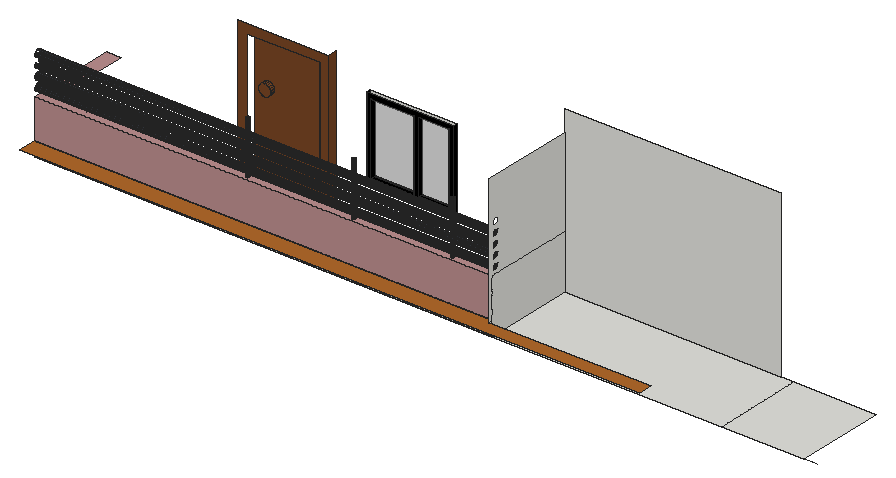
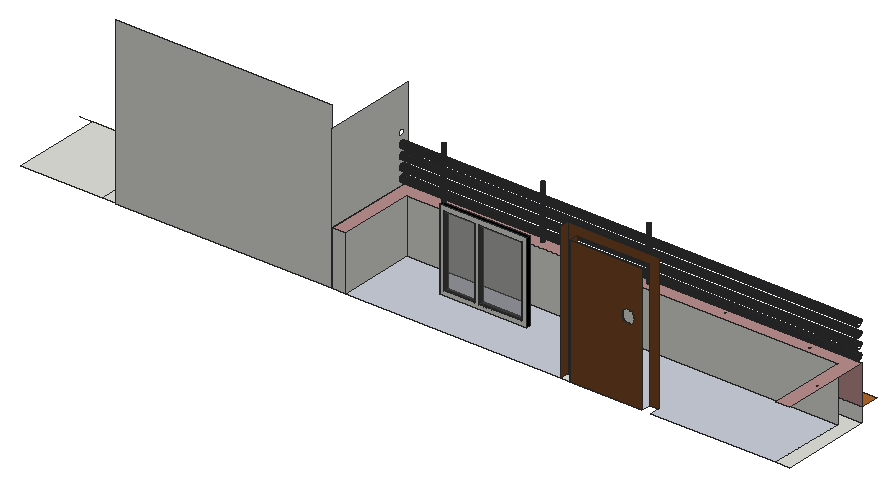
# SketchUp Ruby script. Lengths in inches.
U = 1.inch
M = Sketchup.active_model
def pt(a) = Geom::Point3d.new(a.map { |v| v * U })
def face(e, loops, mat)
  f = e.add_face(loops[0].map { |a| pt(a) })
  loops[1..].each { |l| e.add_face(l.map { |a| pt(a) }).erase! }
  f.material = f.back_material = mat if mat
  f
end
# faces: each face lists its corners as indices into pts; further lists are holes
def faces(e, pts, list, mat = nil) = list.each { |f| face(e, (f[0].is_a?(Array) ? f : [f]).map { |l| l.map { |i| pts[i] } }, mat) }
# xy, xz, yz: faces in a plane at the given z, y or x. An outline is a flat list of corners, or four numbers for a rectangle; further outlines are holes
def ring(l) = l.size == 4 ? [[l[0], l[1]], [l[2], l[1]], [l[2], l[3]], [l[0], l[3]]] : l.each_slice(2).to_a
def flat(e, list, mat, &to3) = list.each { |f| face(e, (f[0].is_a?(Array) ? f : [f]).map { |l| ring(l).map { |u, v| to3.(u, v) } }, mat) }
def xy(e, z, list, mat = nil) = flat(e, list, mat) { |x, y| [x, y, z] }
def xz(e, y, list, mat = nil) = flat(e, list, mat) { |x, z| [x, y, z] }
def yz(e, x, list, mat = nil) = flat(e, list, mat) { |y, z| [x, y, z] }
def lines(e, pts, list) = list.each { |a, b| e.add_line(pt(pts[a]), pt(pts[b])) }
# prism: a flat outline (further loops are holes) pulled along v
def prism(e, loops, v, mat = nil)
  f = face(e, loops, mat); d = Geom::Vector3d.new(v.map { |x| x * U })
  f.pushpull(f.normal.samedirection?(d) ? d.length : -d.length)
end
def box(e, o, s, mat = nil) = prism(e, [[o, [o[0] + s[0], o[1], o[2]], [o[0] + s[0], o[1] + s[1], o[2]], [o[0], o[1] + s[1], o[2]]]], [0, 0, s[2]], mat)
def at(x, y, z, deg = 0) = Geom::Transformation.translation(pt([x, y, z])) * Geom::Transformation.rotation(ORIGIN, Z_AXIS, deg.degrees)
def axes(o, x, y, z) = Geom::Transformation.new([*x, 0, *y, 0, *z, 0, *pt(o).to_a, 1])
def part(name) = M.definitions.add(name)
# library, detail: a bought-in or finely detailed component or shape, given as its bounding box
def library(name, o, s) = part(name).tap { |d| box(d.entities, o, s) }
def detail(e, o, s) = box(e.add_group.entities, o, s)
def put(e, d, t, mat = nil) = e.add_instance(d, t).tap { |i| i.material = mat if mat }
def group(e, t, mat = nil) = e.add_group.tap { |g| g.transformation = t; g.material = mat if mat }.entities
root = M.entities
M.materials.add("[0119_RosyBrown]").color = [188, 143, 143]
M.materials.add("[0137_Black]").color = [0, 0, 0]
M.materials.add("[Formica Laminate Dark]").color = [50, 53, 60]
M.materials.add("[Marble Carrara Floor Tile]").color = [204, 208, 219]
M.materials.add("[Translucent Glass Gray]").color = [128, 128, 128]
M.materials["[Translucent Glass Gray]"].alpha = 0.5
M.materials.add("[Wood Bamboo]").color = [177, 105, 43]
M.materials.add("[Wood Veneer 01]").color = [120, 70, 37]
xy(root,370.9,[[3.53,201.0625,3.53,261.0625,12.53,261.0625,12.53,210.0625,298.22,210.0625,298.22,261.0625,307.22,261.0625,307.22,201.0625],[307.22,201.0625,459.59,261.0625],[459.59,201.0625,514.15,261.0625],[149.3,255.0625,155.3,261.0625]])
xy(root,370.9,[[12.53,210.0625,298.22,210.0625,298.22,261.0625,155.3,261.0625,155.3,255.0625,149.3,255.0625,149.3,261.0625,101.3,261.0625,101.3,255.0625,95.3,255.0625,95.3,261.0625,12.53,261.0625]],"[Marble Carrara Floor Tile]")
xy(root,380.59,[[3.53,189.0625,414.72,189.0625,414.72,198.0625,307.22,198.0625,307.22,201.0625,3.53,201.0625]],"[Wood Bamboo]")
xy(root,392.51,[[178.09,258.0625,235.97,261.0625]])
xy(root,395.51,[[181.09,258.0625,209.84,261.0625],[212.72,258.0625,232.97,261.0625]],"[0137_Black]")
xy(root,406.9,[[142.52,203.04,142.26,203.07,142.02,203.17,141.81,203.33,141.65,203.54,141.55,203.78,141.52,204.04,141.55,204.3,141.65,204.54,141.81,204.75,142.02,204.91,142.26,205.01,142.52,205.04,142.78,205.01,143.02,204.91,143.22,204.75,143.38,204.54,143.48,204.3,143.52,204.04,143.48,203.78,143.38,203.54,143.22,203.33,143.02,203.17,142.78,203.07],[212.89,203.04,212.63,203.07,212.39,203.17,212.18,203.33,212.03,203.54,211.93,203.78,211.89,204.04,211.93,204.3,212.03,204.54,212.18,204.75,212.39,204.91,212.63,205.01,212.89,205.04,213.15,205.01,213.39,204.91,213.6,204.75,213.76,204.54,213.86,204.3,213.89,204.04,213.86,203.78,213.76,203.54,213.6,203.33,213.39,203.17,213.15,203.07]])
xy(root,406.9,[[[3.53,201.0625,307.22,201.0625,307.22,261.0625,298.22,261.0625,298.22,210.0625,12.53,210.0625,12.53,261.0625,3.53,261.0625],[34.52,204.5,34.26,204.53,34.02,204.63,33.82,204.79,33.66,205,33.56,205.24,33.52,205.5,33.56,205.76,33.66,206,33.82,206.21,34.02,206.37,34.26,206.47,34.52,206.5,34.78,206.47,35.02,206.37,35.23,206.21,35.39,206,35.49,205.76,35.52,205.5,35.49,205.24,35.39,205,35.23,204.79,35.02,204.63,34.78,204.53],[91.52,203.04,91.26,203.07,91.02,203.17,90.81,203.33,90.65,203.54,90.55,203.78,90.52,204.04,90.55,204.3,90.65,204.54,90.81,204.75,91.02,204.91,91.26,205.01,91.52,205.04,91.78,205.01,92.02,204.91,92.22,204.75,92.38,204.54,92.48,204.3,92.52,204.04,92.48,203.78,92.38,203.54,92.22,203.33,92.02,203.17,91.78,203.07],[142.52,203.04,142.26,203.07,142.02,203.17,141.81,203.33,141.65,203.54,141.55,203.78,141.52,204.04,141.55,204.3,141.65,204.54,141.81,204.75,142.02,204.91,142.26,205.01,142.52,205.04,142.78,205.01,143.02,204.91,143.22,204.75,143.38,204.54,143.48,204.3,143.52,204.04,143.48,203.78,143.38,203.54,143.22,203.33,143.02,203.17,142.78,203.07],[212.89,203.04,212.63,203.07,212.39,203.17,212.18,203.33,212.03,203.54,211.93,203.78,211.89,204.04,211.93,204.3,212.03,204.54,212.18,204.75,212.39,204.91,212.63,205.01,212.89,205.04,213.15,205.01,213.39,204.91,213.6,204.75,213.76,204.54,213.86,204.3,213.89,204.04,213.86,203.78,213.76,203.54,213.6,203.33,213.39,203.17,213.15,203.07],[278.52,203.04,278.26,203.07,278.02,203.17,277.81,203.33,277.65,203.54,277.55,203.78,277.52,204.04,277.55,204.3,277.65,204.54,277.81,204.75,278.02,204.91,278.26,205.01,278.52,205.04,278.78,205.01,279.02,204.91,279.22,204.75,279.38,204.54,279.48,204.3,279.52,204.04,279.48,203.78,279.38,203.54,279.22,203.33,279.02,203.17,278.78,203.07],[6.47,233.53,6.21,233.57,5.97,233.67,5.76,233.83,5.6,234.03,5.5,234.28,5.47,234.53,5.5,234.79,5.6,235.03,5.76,235.24,5.97,235.4,6.21,235.5,6.47,235.53,6.73,235.5,6.97,235.4,7.17,235.24,7.33,235.03,7.43,234.79,7.47,234.53,7.43,234.28,7.33,234.03,7.17,233.83,6.97,233.67,6.73,233.57]]],"[0119_RosyBrown]")
xz(root,201.0625,[[3.53,370.9,307.22,380.59]])
xz(root,201.0625,[[3.53,380.59,307.22,406.9]],"[0119_RosyBrown]")
xz(root,210.0625,[[12.53,370.9,298.22,406.9]])
xz(root,255.0625,[[95.3,370.9,101.3,370.9,101.3,454.9,149.3,454.9,149.3,370.9,155.3,370.9,155.3,460.9,95.3,460.9]],"[Wood Veneer 01]")
xz(root,258.0625,[[[178.09,392.51,235.97,446.01],[181.09,395.51,209.84,443.01],[212.72,395.51,232.97,443.01]]],"[0137_Black]")
xz(root,258.0625,[[110.53,419.27,111.5625,419.4,112.53,419.8,113.36,420.4375,113.99,421.27,114.39,422.23,114.53,423.27,114.39,424.3,113.99,425.27,113.36,426.09,112.53,426.73,111.5625,427.13,110.53,427.27,109.49,427.13,108.53,426.73,107.7,426.09,107.0625,425.27,106.66,424.3,106.53,423.27,106.66,422.23,107.0625,421.27,107.7,420.4375,108.53,419.8,109.49,419.4]],"[Wood Veneer 01]")
xz(root,261.0625,[[298.22,370.9,307.22,406.9],[307.22,370.9,450.59,480],[[178.09,392.51,235.97,446.01],[181.09,395.51,209.84,443.01],[212.72,395.51,232.97,443.01]],[110.53,419.27,109.49,419.4,108.53,419.8,107.7,420.4375,107.0625,421.27,106.66,422.23,106.53,423.27,106.66,424.3,107.0625,425.27,107.7,426.09,108.53,426.73,109.49,427.13,110.53,427.27,111.5625,427.13,112.53,426.73,113.36,426.09,113.99,425.27,114.39,424.3,114.53,423.27,114.39,422.23,113.99,421.27,113.36,420.4375,112.53,419.8,111.5625,419.4]])
xz(root,261.0625,[[181.09,395.51,209.84,443.01],[212.72,395.51,232.97,443.01]],"[Translucent Glass Gray]")
xz(root,261.0625,[[[101.3,370.9,149.3,454.9],[110.53,419.27,109.49,419.4,108.53,419.8,107.7,420.4375,107.0625,421.27,106.66,422.23,106.53,423.27,106.66,424.3,107.0625,425.27,107.7,426.09,108.53,426.73,109.49,427.13,110.53,427.27,111.5625,427.13,112.53,426.73,113.36,426.09,113.99,425.27,114.39,424.3,114.53,423.27,114.39,422.23,113.99,421.27,113.36,420.4375,112.53,419.8,111.5625,419.4]]],"[Wood Veneer 01]")
yz(root,149.3,[[255.0625,370.9,261.0625,454.9]],"[Wood Veneer 01]")
yz(root,155.3,[[255.0625,370.9,261.0625,460.9]],"[Wood Veneer 01]")
yz(root,178.09,[[258.0625,392.51,261.0625,446.01]],"[0137_Black]")
yz(root,181.09,[[258.0625,395.51,261.0625,443.01]],"[0137_Black]")
yz(root,209.84,[[258.0625,395.51,261.0625,443.01]],"[0137_Black]")
yz(root,212.72,[[258.0625,395.51,261.0625,443.01]],"[0137_Black]")
yz(root,232.97,[[258.0625,395.51,261.0625,443.01]],"[0137_Black]")
yz(root,235.97,[[258.0625,392.51,261.0625,446.01]],"[0137_Black]")
yz(root,298.22,[[210.0625,370.9,261.0625,406.9]])
yz(root,307.22,[[201.0625,370.9,261.0625,406.9],[[198.0625,380.59,198.0625,465.86,261.0625,465.86,261.0625,406.9,201.0625,406.9,201.0625,380.59],[203.51,409.28,204.08,409.36,204.6,409.58,205.06,409.92,205.41,410.375,205.625,410.9,205.7,411.47,205.625,412.04,205.41,412.5625,205.06,413.02,204.6,413.36,204.08,413.58,203.51,413.66,202.94,413.58,202.42,413.36,201.96,413.02,201.62,412.5625,201.4,412.04,201.32,411.47,201.4,410.9,201.62,410.375,201.96,409.92,202.42,409.58,202.94,409.36],[203.51,416.03,204.08,416.11,204.6,416.33,205.06,416.67,205.41,417.125,205.625,417.65,205.7,418.22,205.625,418.79,205.41,419.3125,205.06,419.77,204.6,420.11,204.08,420.33,203.51,420.41,202.94,420.33,202.42,420.11,201.96,419.77,201.62,419.3125,201.4,418.79,201.32,418.22,201.4,417.65,201.62,417.125,201.96,416.67,202.42,416.33,202.94,416.11],[203.51,422.78,204.08,422.86,204.6,423.08,205.06,423.42,205.41,423.875,205.625,424.4,205.7,424.97,205.625,425.54,205.41,426.0625,205.06,426.52,204.6,426.86,204.08,427.08,203.51,427.16,202.94,427.08,202.42,426.86,201.96,426.52,201.62,426.0625,201.4,425.54,201.32,424.97,201.4,424.4,201.62,423.875,201.96,423.42,202.42,423.08,202.94,422.86],[203.51,429.53,204.08,429.61,204.6,429.83,205.06,430.17,205.41,430.625,205.625,431.15,205.7,431.72,205.625,432.29,205.41,432.8125,205.06,433.27,204.6,433.61,204.08,433.83,203.51,433.91,202.94,433.83,202.42,433.61,201.96,433.27,201.62,432.8125,201.4,432.29,201.32,431.72,201.4,431.15,201.62,430.625,201.96,430.17,202.42,429.83,202.94,429.61],[203.51,436.28,204.08,436.36,204.6,436.58,205.06,436.92,205.41,437.375,205.625,437.9,205.7,438.47,205.625,439.04,205.41,439.5625,205.06,440.02,204.6,440.36,204.08,440.58,203.51,440.66,202.94,440.58,202.42,440.36,201.96,440.02,201.62,439.5625,201.4,439.04,201.32,438.47,201.4,437.9,201.62,437.375,201.96,436.92,202.42,436.58,202.94,436.36]]])
p = [[142.26,203.07,406.9],[142.52,203.04,406.9],[142.52,203.04,442.09],[142.26,203.07,442.09],[142.78,203.07,406.9],[142.78,203.07,442.09],
  [212.63,203.07,406.9],[212.89,203.04,406.9],[212.89,203.04,442.09],[212.63,203.07,442.09],[213.15,203.07,406.9],[213.15,203.07,442.09],
  [278.26,203.07,406.9],[278.52,203.04,406.9],[278.52,203.04,442.09],[278.26,203.07,442.09],[278.78,203.07,406.9],[278.78,203.07,442.09],
  [142.02,203.17,406.9],[142.02,203.17,442.09],[143.02,203.17,406.9],[143.02,203.17,442.09],[212.39,203.17,406.9],[212.39,203.17,442.09],
  [213.39,203.17,406.9],[213.39,203.17,442.09],[278.02,203.17,406.9],[278.02,203.17,442.09],[279.02,203.17,406.9],[279.02,203.17,442.09],
  [141.81,203.33,406.9],[141.81,203.33,442.09],[143.22,203.33,406.9],[143.22,203.33,442.09],[212.18,203.33,406.9],[212.18,203.33,442.09],
  [213.6,203.33,406.9],[213.6,203.33,442.09],[277.81,203.33,406.9],[277.81,203.33,442.09],[279.22,203.33,406.9],[279.22,203.33,442.09],
  [141.65,203.54,406.9],[141.65,203.54,442.09],[143.38,203.54,406.9],[143.38,203.54,442.09],[212.03,203.54,406.9],[212.03,203.54,442.09],
  [213.76,203.54,406.9],[213.76,203.54,442.09],[277.65,203.54,406.9],[277.65,203.54,442.09],[279.38,203.54,406.9],[279.38,203.54,442.09],
  [141.55,203.78,406.9],[141.55,203.78,442.09],[143.48,203.78,406.9],[143.48,203.78,442.09],[211.93,203.78,406.9],[211.93,203.78,442.09],
  [213.86,203.78,406.9],[213.86,203.78,442.09],[277.55,203.78,406.9],[277.55,203.78,442.09],[279.48,203.78,406.9],[279.48,203.78,442.09],
  [141.52,204.04,406.9],[141.52,204.04,442.09],[143.52,204.04,406.9],[143.52,204.04,442.09],[211.89,204.04,406.9],[211.89,204.04,442.09],
  [213.89,204.04,406.9],[213.89,204.04,442.09],[277.52,204.04,406.9],[277.52,204.04,442.09],[279.52,204.04,406.9],[279.52,204.04,442.09],
  [141.55,204.3,406.9],[141.55,204.3,442.09],[143.48,204.3,406.9],[143.48,204.3,442.09],[211.93,204.3,406.9],[211.93,204.3,442.09],
  [213.86,204.3,406.9],[213.86,204.3,442.09],[277.55,204.3,406.9],[277.55,204.3,442.09],[279.48,204.3,406.9],[279.48,204.3,442.09],
  [141.65,204.54,406.9],[141.65,204.54,442.09],[143.38,204.54,406.9],[143.38,204.54,442.09],[212.03,204.54,406.9],[212.03,204.54,442.09],
  [213.76,204.54,406.9],[213.76,204.54,442.09],[277.65,204.54,406.9],[277.65,204.54,442.09],[279.38,204.54,406.9],[279.38,204.54,442.09],
  [141.81,204.75,406.9],[141.81,204.75,442.09],[143.22,204.75,406.9],[143.22,204.75,442.09],[212.18,204.75,406.9],[212.18,204.75,442.09],
  [213.6,204.75,406.9],[213.6,204.75,442.09],[277.81,204.75,406.9],[277.81,204.75,442.09],[279.22,204.75,406.9],[279.22,204.75,442.09],
  [142.02,204.91,406.9],[142.02,204.91,442.09],[143.02,204.91,406.9],[143.02,204.91,442.09],[212.39,204.91,406.9],[212.39,204.91,442.09],
  [213.39,204.91,406.9],[213.39,204.91,442.09],[278.02,204.91,406.9],[278.02,204.91,442.09],[279.02,204.91,406.9],[279.02,204.91,442.09],
  [142.26,205.01,406.9],[142.26,205.01,442.09],[142.78,205.01,406.9],[142.78,205.01,442.09],[212.63,205.01,406.9],[212.63,205.01,442.09],
  [213.15,205.01,406.9],[213.15,205.01,442.09],[278.26,205.01,406.9],[278.26,205.01,442.09],[278.78,205.01,406.9],[278.78,205.01,442.09],
  [142.52,205.04,406.9],[142.52,205.04,442.09],[212.89,205.04,406.9],[212.89,205.04,442.09],[278.52,205.04,406.9],[278.52,205.04,442.09],
  [307.22,203.51,409.28],[307.22,202.94,409.36],[3.53,202.94,409.36],[3.53,203.51,409.28],[307.22,204.08,409.36],[3.53,204.08,409.36],
  [307.22,204.6,409.58],[3.53,204.6,409.58],[307.22,205.06,409.92],[3.53,205.06,409.92],[307.22,201.96,409.92],[307.22,201.62,410.375],
  [3.53,201.62,410.375],[3.53,201.96,409.92],[307.22,205.41,410.375],[3.53,205.41,410.375],[307.22,201.4,410.9],[3.53,201.4,410.9],
  [307.22,205.625,410.9],[3.53,205.625,410.9],[307.22,201.32,411.47],[3.53,201.32,411.47],[307.22,205.7,411.47],[3.53,205.7,411.47],
  [307.22,201.4,412.04],[3.53,201.4,412.04],[307.22,205.625,412.04],[3.53,205.625,412.04],[307.22,201.62,412.5625],[3.53,201.62,412.5625],
  [307.22,205.41,412.5625],[3.53,205.41,412.5625],[307.22,201.96,413.02],[3.53,201.96,413.02],[307.22,205.06,413.02],[3.53,205.06,413.02],
  [307.22,202.42,413.36],[3.53,202.42,413.36],[307.22,204.6,413.36],[3.53,204.6,413.36],[307.22,202.94,413.58],[3.53,202.94,413.58],
  [307.22,204.08,413.58],[3.53,204.08,413.58],[307.22,203.51,413.66],[3.53,203.51,413.66],[307.22,203.51,416.03],[307.22,202.94,416.11],
  [3.53,202.94,416.11],[3.53,203.51,416.03],[307.22,204.08,416.11],[3.53,204.08,416.11],[307.22,204.6,416.33],[3.53,204.6,416.33],
  [307.22,205.06,416.67],[3.53,205.06,416.67],[307.22,201.96,416.67],[307.22,201.62,417.125],[3.53,201.62,417.125],[3.53,201.96,416.67],
  [307.22,205.41,417.125],[3.53,205.41,417.125],[307.22,201.4,417.65],[3.53,201.4,417.65],[307.22,205.625,417.65],[3.53,205.55,417.48],
  [3.53,205.625,417.65],[307.22,201.32,418.22],[3.53,201.32,418.22],[307.22,205.7,418.22],[3.53,205.7,418.22],[307.22,201.4,418.79],
  [3.53,201.4,418.79],[307.22,205.625,418.79],[3.53,205.65,418.61],[3.53,205.625,418.79],[307.22,201.62,419.3125],[3.53,201.62,419.3125],
  [307.22,205.41,419.3125],[3.53,205.41,419.3125],[307.22,201.96,419.77],[3.53,201.96,419.77],[307.22,205.06,419.77],[3.53,205.06,419.77],
  [109.49,261.0625,419.4],[110.53,261.0625,419.27],[110.53,258.0625,419.27],[109.49,258.0625,419.4],[111.5625,261.0625,419.4],[111.5625,258.0625,419.4],
  [108.53,261.0625,419.8],[108.53,258.0625,419.8],[112.53,261.0625,419.8],[112.53,258.0625,419.8],[307.22,204.6,420.11],[3.53,204.6,420.11],
  [107.7,261.0625,420.4375],[107.7,258.0625,420.4375],[113.36,261.0625,420.4375],[113.36,258.0625,420.4375],[307.22,204.08,420.33],[3.53,204.08,420.33],
  [307.22,202.94,420.33],[307.22,203.51,420.41],[3.53,203.51,420.41],[3.53,202.94,420.33],[113.99,261.0625,421.27],[113.99,258.0625,421.27],
  [114.39,261.0625,422.23],[114.39,258.0625,422.23],[114.53,261.0625,423.27],[114.53,258.0625,423.27],[307.22,203.51,422.78],[307.22,202.94,422.86],
  [5.64,202.94,422.86],[3.53,202.94,422.86],[3.53,203.51,422.78],[307.22,204.08,422.86],[3.53,204.08,422.86],[5.64,204.08,422.86],
  [307.22,204.6,423.08],[3.53,204.6,423.08],[307.22,205.06,423.42],[3.53,205.06,423.42],[114.39,261.0625,424.3],[114.39,258.0625,424.3],
  [307.22,201.96,423.42],[307.22,201.62,423.875],[3.53,201.62,423.875],[3.53,201.96,423.42],[307.22,205.41,423.875],[3.53,205.41,423.875],
  [307.22,201.4,424.4],[3.53,201.4,424.4],[307.22,205.625,424.4],[3.53,205.625,424.4],[113.99,261.0625,425.27],[113.99,258.0625,425.27],
  [307.22,201.32,424.97],[3.53,201.32,424.97],[307.22,205.7,424.97],[3.53,205.63,424.48],[3.53,205.7,424.97],[307.22,201.4,425.54],
  [3.53,201.4,425.54],[307.22,205.625,425.54],[3.53,205.625,425.54],[107.7,261.0625,426.09],[107.0625,261.0625,425.27],[107.0625,258.0625,425.27],
  [107.7,258.0625,426.09],[113.36,261.0625,426.09],[113.36,258.0625,426.09],[307.22,201.62,426.0625],[3.53,201.62,426.0625],[307.22,205.41,426.0625],
  [3.53,205.59,425.61],[3.53,205.41,426.0625],[307.22,201.96,426.52],[3.53,201.96,426.52],[307.22,205.06,426.52],[3.53,205.06,426.52],
  [108.53,261.0625,426.73],[108.53,258.0625,426.73],[112.53,261.0625,426.73],[112.53,258.0625,426.73],[307.22,204.6,426.86],[3.53,204.6,426.86],
  [109.49,261.0625,427.13],[109.49,258.0625,427.13],[111.5625,261.0625,427.13],[111.5625,258.0625,427.13],[307.22,204.08,427.08],[3.53,204.08,427.08],
  [110.53,261.0625,427.27],[110.53,258.0625,427.27],[307.22,203.51,429.53],[307.22,202.94,429.61],[3.53,202.94,429.61],[3.53,203.51,429.53],
  [307.22,204.08,429.61],[3.53,204.08,429.61],[307.22,204.6,429.83],[3.53,204.6,429.83],[307.22,205.06,430.17],[3.53,205.06,430.17],
  [307.22,201.96,430.17],[307.22,201.62,430.625],[3.53,201.62,430.625],[3.53,201.96,430.17],[307.22,205.41,430.625],[3.53,205.41,430.625],
  [307.22,201.4,431.15],[3.53,201.4,431.15],[307.22,205.625,431.15],[3.53,205.625,431.15],[307.22,201.32,431.72],[3.53,201.32,431.72],
  [307.22,205.7,431.72],[3.53,205.64,431.29],[3.53,205.7,431.72],[307.22,201.4,432.29],[3.53,201.4,432.29],[307.22,205.625,432.29],
  [3.53,205.625,432.29],[307.22,201.62,432.8125],[3.53,201.62,432.8125],[307.22,205.41,432.8125],[3.53,205.57,432.42],[3.53,205.41,432.8125],
  [307.22,201.96,433.27],[3.53,201.96,433.27],[307.22,205.06,433.27],[3.53,205.06,433.27],[307.22,204.6,433.61],[3.53,204.6,433.61],
  [307.22,204.08,433.83],[3.53,204.08,433.83],[307.22,202.94,433.83],[307.22,203.51,433.91],[3.53,203.51,433.91],[3.53,202.94,433.83],
  [514.15,201.0625,370.9],[522.97,201.0625,370.9]]
faces(root,p,[[0,1,2,3],[1,4,5,2],[6,7,8,9],[7,10,11,8],[12,13,14,15],[13,16,17,14],[18,0,3,19],[4,20,21,5],
  [22,6,9,23],[10,24,25,11],[26,12,15,27],[16,28,29,17],[30,18,19,31],[20,32,33,21],[34,22,23,35],[24,36,37,25],
  [38,26,27,39],[28,40,41,29],[42,30,31,43],[32,44,45,33],[46,34,35,47],[36,48,49,37],[50,38,39,51],[40,52,53,41],
  [54,42,43,55],[44,56,57,45],[58,46,47,59],[48,60,61,49],[62,50,51,63],[52,64,65,53],[66,54,55,67],[56,68,69,57],
  [70,58,59,71],[60,72,73,61],[74,62,63,75],[64,76,77,65],[78,66,67,79],[68,80,81,69],[82,70,71,83],[72,84,85,73],
  [86,74,75,87],[76,88,89,77],[90,78,79,91],[80,92,93,81],[94,82,83,95],[84,96,97,85],[98,86,87,99],[88,100,101,89],
  [102,90,91,103],[92,104,105,93],[106,94,95,107],[96,108,109,97],[110,98,99,111],[100,112,113,101],[114,102,103,115],[104,116,117,105],
  [118,106,107,119],[108,120,121,109],[122,110,111,123],[112,124,125,113],[126,114,115,127],[116,128,129,117],[130,118,119,131],[120,132,133,121],
  [134,122,123,135],[124,136,137,125],[138,126,127,139],[128,138,139,129],[140,130,131,141],[132,140,141,133],[142,134,135,143],[136,142,143,137],
  [144,145,146,147],[148,144,147,149],[150,148,149,151],[152,150,151,153],[154,155,156,157],[158,152,153,159],[155,160,161,156],[162,158,159,163],
  [160,164,165,161],[166,162,163,167],[164,168,169,165],[170,166,167,171],[168,172,173,169],[174,170,171,175],[172,176,177,173],[178,174,175,179],
  [176,180,181,177],[182,178,179,183],[180,184,185,181],[186,182,183,187],[184,188,189,185],[188,186,187,189],[190,191,192,193],[194,190,193,195],
  [196,194,195,197],[198,196,197,199],[200,201,202,203],[204,198,199,205],[201,206,207,202],[208,204,205,209,210],[206,211,212,207],[213,208,210,214],
  [211,215,216,212],[217,213,214,218,219],[215,220,221,216],[222,217,219,223],[220,224,225,221],[226,222,223,227],[238,226,227,239],[244,238,239,245],
  [246,247,248,249],[247,244,245,248],[256,257,258,259,260],[261,256,260,262,263],[264,261,263,262,265],[266,264,265,267],[270,271,272,273],[274,266,267,275],
  [271,276,277,272],[278,274,275,279],[276,282,283,277],[284,278,279,285,286],[282,287,288,283],[289,284,286,290],[287,297,298,288],[299,289,290,300,301],
  [297,302,303,298],[304,299,301,305],[310,304,305,311],[316,310,311,317],[320,321,322,323],[324,320,323,325],[326,324,325,327],[328,326,327,329],
  [330,331,332,333],[334,328,329,335],[331,336,337,332],[338,334,335,339],[336,340,341,337],[342,338,339,343,344],[340,345,346,341],[347,342,344,348],
  [345,349,350,346],[351,347,348,352,353],[349,354,355,350],[356,351,353,357],[358,356,357,359],[360,358,359,361],[362,363,364,365],[363,360,361,364]],"[Formica Laminate Dark]")
faces(root,p,[[228,229,230,231],[229,232,233,230],[234,228,231,235],[232,236,237,233],[240,234,235,241],[236,242,243,237],[242,250,251,243],[250,252,253,251],
  [252,254,255,253],[254,268,269,255],[268,280,281,269],[291,292,293,294],[280,295,296,281],[306,291,294,307],[295,308,309,296],[312,306,307,313],
  [308,314,315,309],[318,312,313,319],[314,318,319,315]],"[Wood Veneer 01]")
lines(root,p,[[366,367]])
